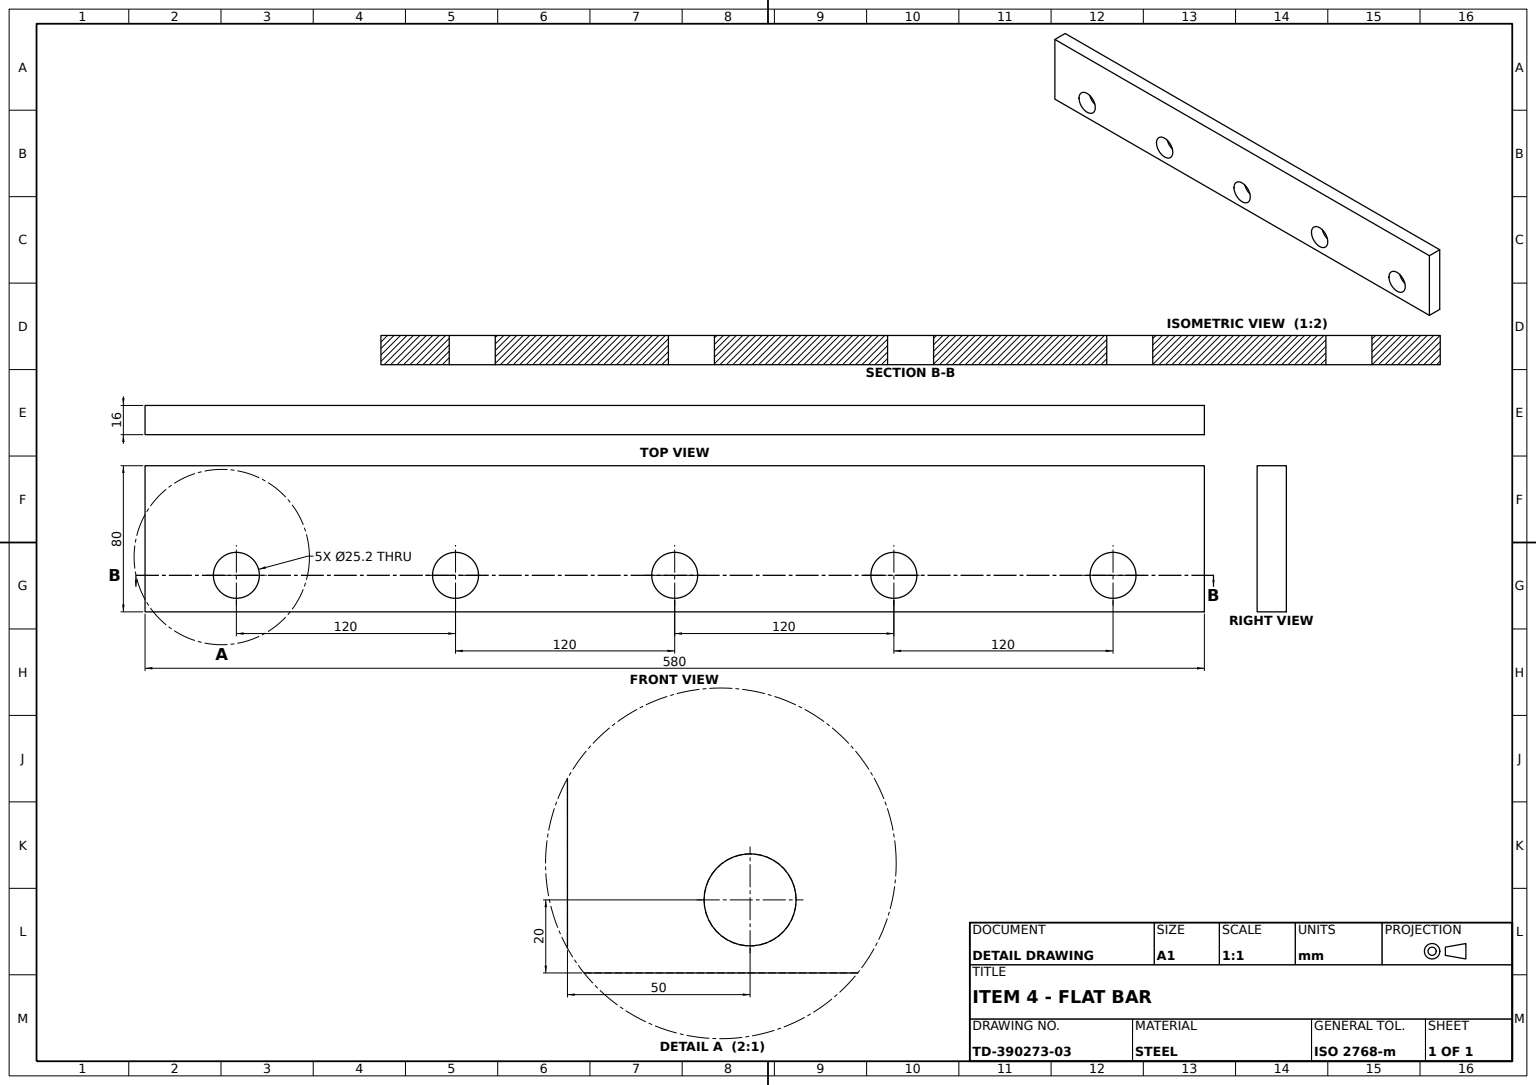
ISO-10303-21;
HEADER;
FILE_DESCRIPTION((''),'2;1');
FILE_NAME('','',(''),(''),'','','');
FILE_SCHEMA(('AUTOMOTIVE_DESIGN'));
ENDSEC;
DATA;
#1=APPLICATION_CONTEXT('');
#2=PRODUCT_CONTEXT('',#1,'mechanical');
#3=PRODUCT('','','',(#2));
#4=PRODUCT_DEFINITION_FORMATION('','',#3);
#5=PRODUCT_DEFINITION_CONTEXT('',#1,'design');
#6=PRODUCT_DEFINITION('','',#4,#5);
#7=PRODUCT_DEFINITION_SHAPE('','',#6);
#8=(LENGTH_UNIT()NAMED_UNIT(*)SI_UNIT(.MILLI.,.METRE.));
#9=(NAMED_UNIT(*)PLANE_ANGLE_UNIT()SI_UNIT($,.RADIAN.));
#10=(NAMED_UNIT(*)SI_UNIT($,.STERADIAN.)SOLID_ANGLE_UNIT());
#11=UNCERTAINTY_MEASURE_WITH_UNIT(LENGTH_MEASURE(1.E-05),#8,'distance_accuracy_value','');
#12=(GEOMETRIC_REPRESENTATION_CONTEXT(3)GLOBAL_UNCERTAINTY_ASSIGNED_CONTEXT((#11))GLOBAL_UNIT_ASSIGNED_CONTEXT((#8,#9,#10))REPRESENTATION_CONTEXT('',''));
#13=CARTESIAN_POINT('',(12.6,-20.,0.));
#14=VERTEX_POINT('',#13);
#15=CARTESIAN_POINT('',(12.6,-20.,16.));
#16=VERTEX_POINT('',#15);
#17=CARTESIAN_POINT('',(12.6,-20.,-10.));
#18=DIRECTION('',(0.,0.,1.));
#19=VECTOR('',#18,1000.);
#20=LINE('',#17,#19);
#21=EDGE_CURVE('',#14,#16,#20,.T.);
#22=ORIENTED_EDGE('',*,*,#21,.T.);
#23=CARTESIAN_POINT('',(-12.6,-20.,16.));
#24=VERTEX_POINT('',#23);
#25=CARTESIAN_POINT('',(0.,-20.,16.));
#26=DIRECTION('',(1.,0.,0.));
#27=AXIS2_PLACEMENT_3D('',#25,#18,#26);
#28=CIRCLE('',#27,12.6);
#29=EDGE_CURVE('',#16,#24,#28,.T.);
#30=ORIENTED_EDGE('',*,*,#29,.T.);
#31=CARTESIAN_POINT('',(-12.6,-20.,0.));
#32=VERTEX_POINT('',#31);
#33=CARTESIAN_POINT('',(-12.6,-20.,-10.));
#34=LINE('',#33,#19);
#35=EDGE_CURVE('',#32,#24,#34,.T.);
#36=ORIENTED_EDGE('',*,*,#35,.F.);
#37=CARTESIAN_POINT('',(0.,-20.,0.));
#38=AXIS2_PLACEMENT_3D('',#37,#18,#26);
#39=CIRCLE('',#38,12.6);
#40=EDGE_CURVE('',#14,#32,#39,.T.);
#41=ORIENTED_EDGE('',*,*,#40,.F.);
#42=EDGE_LOOP('',(#22,#30,#36,#41));
#43=FACE_OUTER_BOUND('',#42,.T.);
#44=CARTESIAN_POINT('',(0.,-20.,-10.));
#45=AXIS2_PLACEMENT_3D('',#44,#18,#26);
#46=CYLINDRICAL_SURFACE('',#45,12.6);
#47=ADVANCED_FACE('',(#43),#46,.F.);
#48=CARTESIAN_POINT('',(-252.6,-20.,0.));
#49=VERTEX_POINT('',#48);
#50=CARTESIAN_POINT('',(-227.4,-20.,0.));
#51=VERTEX_POINT('',#50);
#52=CARTESIAN_POINT('',(-240.,-20.,0.));
#53=AXIS2_PLACEMENT_3D('',#52,#18,#26);
#54=CIRCLE('',#53,12.6);
#55=EDGE_CURVE('',#49,#51,#54,.T.);
#56=ORIENTED_EDGE('',*,*,#55,.T.);
#57=EDGE_CURVE('',#51,#49,#54,.T.);
#58=ORIENTED_EDGE('',*,*,#57,.T.);
#59=EDGE_LOOP('',(#56,#58));
#60=FACE_BOUND('',#59,.T.);
#61=CARTESIAN_POINT('',(-290.,40.,0.));
#62=VERTEX_POINT('',#61);
#63=CARTESIAN_POINT('',(-290.,-40.,0.));
#64=VERTEX_POINT('',#63);
#65=DIRECTION('',(0.,-1.,0.));
#66=VECTOR('',#65,1000.);
#67=LINE('',#61,#66);
#68=EDGE_CURVE('',#62,#64,#67,.T.);
#69=ORIENTED_EDGE('',*,*,#68,.F.);
#70=CARTESIAN_POINT('',(290.,40.,0.));
#71=VERTEX_POINT('',#70);
#72=DIRECTION('',(-1.,0.,0.));
#73=VECTOR('',#72,1000.);
#74=LINE('',#61,#73);
#75=EDGE_CURVE('',#71,#62,#74,.T.);
#76=ORIENTED_EDGE('',*,*,#75,.F.);
#77=CARTESIAN_POINT('',(290.,-40.,0.));
#78=VERTEX_POINT('',#77);
#79=DIRECTION('',(0.,1.,0.));
#80=VECTOR('',#79,1000.);
#81=LINE('',#70,#80);
#82=EDGE_CURVE('',#78,#71,#81,.T.);
#83=ORIENTED_EDGE('',*,*,#82,.F.);
#84=VECTOR('',#26,1000.);
#85=LINE('',#63,#84);
#86=EDGE_CURVE('',#64,#78,#85,.T.);
#87=ORIENTED_EDGE('',*,*,#86,.F.);
#88=EDGE_LOOP('',(#69,#76,#83,#87));
#89=FACE_OUTER_BOUND('',#88,.T.);
#90=CARTESIAN_POINT('',(-107.4,-20.,0.));
#91=VERTEX_POINT('',#90);
#92=CARTESIAN_POINT('',(-132.6,-20.,0.));
#93=VERTEX_POINT('',#92);
#94=CARTESIAN_POINT('',(-120.,-20.,0.));
#95=AXIS2_PLACEMENT_3D('',#94,#18,#26);
#96=CIRCLE('',#95,12.6);
#97=EDGE_CURVE('',#91,#93,#96,.T.);
#98=ORIENTED_EDGE('',*,*,#97,.T.);
#99=EDGE_CURVE('',#93,#91,#96,.T.);
#100=ORIENTED_EDGE('',*,*,#99,.T.);
#101=EDGE_LOOP('',(#98,#100));
#102=FACE_BOUND('',#101,.T.);
#103=CARTESIAN_POINT('',(107.4,-20.,0.));
#104=VERTEX_POINT('',#103);
#105=CARTESIAN_POINT('',(132.6,-20.,0.));
#106=VERTEX_POINT('',#105);
#107=CARTESIAN_POINT('',(120.,-20.,0.));
#108=AXIS2_PLACEMENT_3D('',#107,#18,#26);
#109=CIRCLE('',#108,12.6);
#110=EDGE_CURVE('',#104,#106,#109,.T.);
#111=ORIENTED_EDGE('',*,*,#110,.T.);
#112=EDGE_CURVE('',#106,#104,#109,.T.);
#113=ORIENTED_EDGE('',*,*,#112,.T.);
#114=EDGE_LOOP('',(#111,#113));
#115=FACE_BOUND('',#114,.T.);
#116=EDGE_CURVE('',#32,#14,#39,.T.);
#117=ORIENTED_EDGE('',*,*,#116,.T.);
#118=ORIENTED_EDGE('',*,*,#40,.T.);
#119=EDGE_LOOP('',(#117,#118));
#120=FACE_BOUND('',#119,.T.);
#121=CARTESIAN_POINT('',(252.6,-20.,0.));
#122=VERTEX_POINT('',#121);
#123=CARTESIAN_POINT('',(227.4,-20.,0.));
#124=VERTEX_POINT('',#123);
#125=CARTESIAN_POINT('',(240.,-20.,0.));
#126=AXIS2_PLACEMENT_3D('',#125,#18,#26);
#127=CIRCLE('',#126,12.6);
#128=EDGE_CURVE('',#122,#124,#127,.T.);
#129=ORIENTED_EDGE('',*,*,#128,.T.);
#130=EDGE_CURVE('',#124,#122,#127,.T.);
#131=ORIENTED_EDGE('',*,*,#130,.T.);
#132=EDGE_LOOP('',(#129,#131));
#133=FACE_BOUND('',#132,.T.);
#134=CARTESIAN_POINT('',(0.,0.,0.));
#135=AXIS2_PLACEMENT_3D('',#134,#18,#26);
#136=PLANE('',#135);
#137=ADVANCED_FACE('',(#60,#89,#102,#115,#120,#133),#136,.F.);
#138=CARTESIAN_POINT('',(227.4,-20.,16.));
#139=VERTEX_POINT('',#138);
#140=CARTESIAN_POINT('',(227.4,-20.,-10.));
#141=LINE('',#140,#19);
#142=EDGE_CURVE('',#124,#139,#141,.T.);
#143=ORIENTED_EDGE('',*,*,#142,.F.);
#144=ORIENTED_EDGE('',*,*,#128,.F.);
#145=CARTESIAN_POINT('',(252.6,-20.,16.));
#146=VERTEX_POINT('',#145);
#147=CARTESIAN_POINT('',(252.6,-20.,-10.));
#148=LINE('',#147,#19);
#149=EDGE_CURVE('',#122,#146,#148,.T.);
#150=ORIENTED_EDGE('',*,*,#149,.T.);
#151=CARTESIAN_POINT('',(240.,-20.,16.));
#152=AXIS2_PLACEMENT_3D('',#151,#18,#26);
#153=CIRCLE('',#152,12.6);
#154=EDGE_CURVE('',#146,#139,#153,.T.);
#155=ORIENTED_EDGE('',*,*,#154,.T.);
#156=EDGE_LOOP('',(#143,#144,#150,#155));
#157=FACE_OUTER_BOUND('',#156,.T.);
#158=CARTESIAN_POINT('',(240.,-20.,-10.));
#159=AXIS2_PLACEMENT_3D('',#158,#18,#26);
#160=CYLINDRICAL_SURFACE('',#159,12.6);
#161=ADVANCED_FACE('',(#157),#160,.F.);
#162=ORIENTED_EDGE('',*,*,#116,.F.);
#163=ORIENTED_EDGE('',*,*,#35,.T.);
#164=EDGE_CURVE('',#24,#16,#28,.T.);
#165=ORIENTED_EDGE('',*,*,#164,.T.);
#166=ORIENTED_EDGE('',*,*,#21,.F.);
#167=EDGE_LOOP('',(#162,#163,#165,#166));
#168=FACE_OUTER_BOUND('',#167,.T.);
#169=ADVANCED_FACE('',(#168),#46,.F.);
#170=CARTESIAN_POINT('',(-290.,-40.,16.));
#171=VERTEX_POINT('',#170);
#172=DIRECTION('',(0.,0.,-1.));
#173=VECTOR('',#172,1000.);
#174=LINE('',#170,#173);
#175=EDGE_CURVE('',#171,#64,#174,.T.);
#176=ORIENTED_EDGE('',*,*,#175,.F.);
#177=CARTESIAN_POINT('',(-290.,40.,16.));
#178=VERTEX_POINT('',#177);
#179=LINE('',#177,#66);
#180=EDGE_CURVE('',#178,#171,#179,.T.);
#181=ORIENTED_EDGE('',*,*,#180,.F.);
#182=LINE('',#177,#173);
#183=EDGE_CURVE('',#178,#62,#182,.T.);
#184=ORIENTED_EDGE('',*,*,#183,.T.);
#185=ORIENTED_EDGE('',*,*,#68,.T.);
#186=EDGE_LOOP('',(#176,#181,#184,#185));
#187=FACE_OUTER_BOUND('',#186,.T.);
#188=AXIS2_PLACEMENT_3D('',#177,#26,#172);
#189=PLANE('',#188);
#190=ADVANCED_FACE('',(#187),#189,.F.);
#191=CARTESIAN_POINT('',(-107.4,-20.,16.));
#192=VERTEX_POINT('',#191);
#193=CARTESIAN_POINT('',(-132.6,-20.,16.));
#194=VERTEX_POINT('',#193);
#195=CARTESIAN_POINT('',(-120.,-20.,16.));
#196=AXIS2_PLACEMENT_3D('',#195,#18,#26);
#197=CIRCLE('',#196,12.6);
#198=EDGE_CURVE('',#192,#194,#197,.T.);
#199=ORIENTED_EDGE('',*,*,#198,.T.);
#200=CARTESIAN_POINT('',(-132.6,-20.,-10.));
#201=LINE('',#200,#19);
#202=EDGE_CURVE('',#93,#194,#201,.T.);
#203=ORIENTED_EDGE('',*,*,#202,.F.);
#204=ORIENTED_EDGE('',*,*,#97,.F.);
#205=CARTESIAN_POINT('',(-107.4,-20.,-10.));
#206=LINE('',#205,#19);
#207=EDGE_CURVE('',#91,#192,#206,.T.);
#208=ORIENTED_EDGE('',*,*,#207,.T.);
#209=EDGE_LOOP('',(#199,#203,#204,#208));
#210=FACE_OUTER_BOUND('',#209,.T.);
#211=CARTESIAN_POINT('',(-120.,-20.,-10.));
#212=AXIS2_PLACEMENT_3D('',#211,#18,#26);
#213=CYLINDRICAL_SURFACE('',#212,12.6);
#214=ADVANCED_FACE('',(#210),#213,.F.);
#215=ORIENTED_EDGE('',*,*,#164,.F.);
#216=ORIENTED_EDGE('',*,*,#29,.F.);
#217=EDGE_LOOP('',(#215,#216));
#218=FACE_BOUND('',#217,.T.);
#219=CARTESIAN_POINT('',(-227.4,-20.,16.));
#220=VERTEX_POINT('',#219);
#221=CARTESIAN_POINT('',(-252.6,-20.,16.));
#222=VERTEX_POINT('',#221);
#223=CARTESIAN_POINT('',(-240.,-20.,16.));
#224=AXIS2_PLACEMENT_3D('',#223,#18,#26);
#225=CIRCLE('',#224,12.6);
#226=EDGE_CURVE('',#220,#222,#225,.T.);
#227=ORIENTED_EDGE('',*,*,#226,.F.);
#228=EDGE_CURVE('',#222,#220,#225,.T.);
#229=ORIENTED_EDGE('',*,*,#228,.F.);
#230=EDGE_LOOP('',(#227,#229));
#231=FACE_BOUND('',#230,.T.);
#232=CARTESIAN_POINT('',(107.4,-20.,16.));
#233=VERTEX_POINT('',#232);
#234=CARTESIAN_POINT('',(132.6,-20.,16.));
#235=VERTEX_POINT('',#234);
#236=CARTESIAN_POINT('',(120.,-20.,16.));
#237=AXIS2_PLACEMENT_3D('',#236,#18,#26);
#238=CIRCLE('',#237,12.6);
#239=EDGE_CURVE('',#233,#235,#238,.T.);
#240=ORIENTED_EDGE('',*,*,#239,.F.);
#241=EDGE_CURVE('',#235,#233,#238,.T.);
#242=ORIENTED_EDGE('',*,*,#241,.F.);
#243=EDGE_LOOP('',(#240,#242));
#244=FACE_BOUND('',#243,.T.);
#245=ORIENTED_EDGE('',*,*,#198,.F.);
#246=EDGE_CURVE('',#194,#192,#197,.T.);
#247=ORIENTED_EDGE('',*,*,#246,.F.);
#248=EDGE_LOOP('',(#245,#247));
#249=FACE_BOUND('',#248,.T.);
#250=ORIENTED_EDGE('',*,*,#154,.F.);
#251=EDGE_CURVE('',#139,#146,#153,.T.);
#252=ORIENTED_EDGE('',*,*,#251,.F.);
#253=EDGE_LOOP('',(#250,#252));
#254=FACE_BOUND('',#253,.T.);
#255=ORIENTED_EDGE('',*,*,#180,.T.);
#256=CARTESIAN_POINT('',(290.,-40.,16.));
#257=VERTEX_POINT('',#256);
#258=LINE('',#170,#84);
#259=EDGE_CURVE('',#171,#257,#258,.T.);
#260=ORIENTED_EDGE('',*,*,#259,.T.);
#261=CARTESIAN_POINT('',(290.,40.,16.));
#262=VERTEX_POINT('',#261);
#263=LINE('',#261,#80);
#264=EDGE_CURVE('',#257,#262,#263,.T.);
#265=ORIENTED_EDGE('',*,*,#264,.T.);
#266=LINE('',#177,#73);
#267=EDGE_CURVE('',#262,#178,#266,.T.);
#268=ORIENTED_EDGE('',*,*,#267,.T.);
#269=EDGE_LOOP('',(#255,#260,#265,#268));
#270=FACE_OUTER_BOUND('',#269,.T.);
#271=CARTESIAN_POINT('',(0.,0.,16.));
#272=AXIS2_PLACEMENT_3D('',#271,#18,#26);
#273=PLANE('',#272);
#274=ADVANCED_FACE('',(#218,#231,#244,#249,#254,#270),#273,.T.);
#275=ORIENTED_EDGE('',*,*,#75,.T.);
#276=ORIENTED_EDGE('',*,*,#183,.F.);
#277=ORIENTED_EDGE('',*,*,#267,.F.);
#278=LINE('',#261,#173);
#279=EDGE_CURVE('',#262,#71,#278,.T.);
#280=ORIENTED_EDGE('',*,*,#279,.T.);
#281=EDGE_LOOP('',(#275,#276,#277,#280));
#282=FACE_OUTER_BOUND('',#281,.T.);
#283=AXIS2_PLACEMENT_3D('',#177,#65,#172);
#284=PLANE('',#283);
#285=ADVANCED_FACE('',(#282),#284,.F.);
#286=ORIENTED_EDGE('',*,*,#175,.T.);
#287=ORIENTED_EDGE('',*,*,#86,.T.);
#288=LINE('',#256,#173);
#289=EDGE_CURVE('',#257,#78,#288,.T.);
#290=ORIENTED_EDGE('',*,*,#289,.F.);
#291=ORIENTED_EDGE('',*,*,#259,.F.);
#292=EDGE_LOOP('',(#286,#287,#290,#291));
#293=FACE_OUTER_BOUND('',#292,.T.);
#294=AXIS2_PLACEMENT_3D('',#170,#79,#18);
#295=PLANE('',#294);
#296=ADVANCED_FACE('',(#293),#295,.F.);
#297=ORIENTED_EDGE('',*,*,#279,.F.);
#298=ORIENTED_EDGE('',*,*,#264,.F.);
#299=ORIENTED_EDGE('',*,*,#289,.T.);
#300=ORIENTED_EDGE('',*,*,#82,.T.);
#301=EDGE_LOOP('',(#297,#298,#299,#300));
#302=FACE_OUTER_BOUND('',#301,.T.);
#303=AXIS2_PLACEMENT_3D('',#261,#72,#18);
#304=PLANE('',#303);
#305=ADVANCED_FACE('',(#302),#304,.F.);
#306=ORIENTED_EDGE('',*,*,#226,.T.);
#307=CARTESIAN_POINT('',(-252.6,-20.,-10.));
#308=LINE('',#307,#19);
#309=EDGE_CURVE('',#49,#222,#308,.T.);
#310=ORIENTED_EDGE('',*,*,#309,.F.);
#311=ORIENTED_EDGE('',*,*,#57,.F.);
#312=CARTESIAN_POINT('',(-227.4,-20.,-10.));
#313=LINE('',#312,#19);
#314=EDGE_CURVE('',#51,#220,#313,.T.);
#315=ORIENTED_EDGE('',*,*,#314,.T.);
#316=EDGE_LOOP('',(#306,#310,#311,#315));
#317=FACE_OUTER_BOUND('',#316,.T.);
#318=CARTESIAN_POINT('',(-240.,-20.,-10.));
#319=AXIS2_PLACEMENT_3D('',#318,#18,#26);
#320=CYLINDRICAL_SURFACE('',#319,12.6);
#321=ADVANCED_FACE('',(#317),#320,.F.);
#322=ORIENTED_EDGE('',*,*,#112,.F.);
#323=CARTESIAN_POINT('',(132.6,-20.,-10.));
#324=LINE('',#323,#19);
#325=EDGE_CURVE('',#106,#235,#324,.T.);
#326=ORIENTED_EDGE('',*,*,#325,.T.);
#327=ORIENTED_EDGE('',*,*,#241,.T.);
#328=CARTESIAN_POINT('',(107.4,-20.,-10.));
#329=LINE('',#328,#19);
#330=EDGE_CURVE('',#104,#233,#329,.T.);
#331=ORIENTED_EDGE('',*,*,#330,.F.);
#332=EDGE_LOOP('',(#322,#326,#327,#331));
#333=FACE_OUTER_BOUND('',#332,.T.);
#334=CARTESIAN_POINT('',(120.,-20.,-10.));
#335=AXIS2_PLACEMENT_3D('',#334,#18,#26);
#336=CYLINDRICAL_SURFACE('',#335,12.6);
#337=ADVANCED_FACE('',(#333),#336,.F.);
#338=ORIENTED_EDGE('',*,*,#251,.T.);
#339=ORIENTED_EDGE('',*,*,#149,.F.);
#340=ORIENTED_EDGE('',*,*,#130,.F.);
#341=ORIENTED_EDGE('',*,*,#142,.T.);
#342=EDGE_LOOP('',(#338,#339,#340,#341));
#343=FACE_OUTER_BOUND('',#342,.T.);
#344=ADVANCED_FACE('',(#343),#160,.F.);
#345=ORIENTED_EDGE('',*,*,#314,.F.);
#346=ORIENTED_EDGE('',*,*,#55,.F.);
#347=ORIENTED_EDGE('',*,*,#309,.T.);
#348=ORIENTED_EDGE('',*,*,#228,.T.);
#349=EDGE_LOOP('',(#345,#346,#347,#348));
#350=FACE_OUTER_BOUND('',#349,.T.);
#351=ADVANCED_FACE('',(#350),#320,.F.);
#352=ORIENTED_EDGE('',*,*,#202,.T.);
#353=ORIENTED_EDGE('',*,*,#246,.T.);
#354=ORIENTED_EDGE('',*,*,#207,.F.);
#355=ORIENTED_EDGE('',*,*,#99,.F.);
#356=EDGE_LOOP('',(#352,#353,#354,#355));
#357=FACE_OUTER_BOUND('',#356,.T.);
#358=ADVANCED_FACE('',(#357),#213,.F.);
#359=ORIENTED_EDGE('',*,*,#325,.F.);
#360=ORIENTED_EDGE('',*,*,#110,.F.);
#361=ORIENTED_EDGE('',*,*,#330,.T.);
#362=ORIENTED_EDGE('',*,*,#239,.T.);
#363=EDGE_LOOP('',(#359,#360,#361,#362));
#364=FACE_OUTER_BOUND('',#363,.T.);
#365=ADVANCED_FACE('',(#364),#336,.F.);
#366=CLOSED_SHELL('',(#47,#137,#161,#169,#190,#214,#274,#285,#296,#305,#321,#337,#344,#351,#358,#365));
#367=MANIFOLD_SOLID_BREP('',#366);
#368=ADVANCED_BREP_SHAPE_REPRESENTATION('',(#367),#12);
#369=SHAPE_DEFINITION_REPRESENTATION(#7,#368);
ENDSEC;
END-ISO-10303-21;
